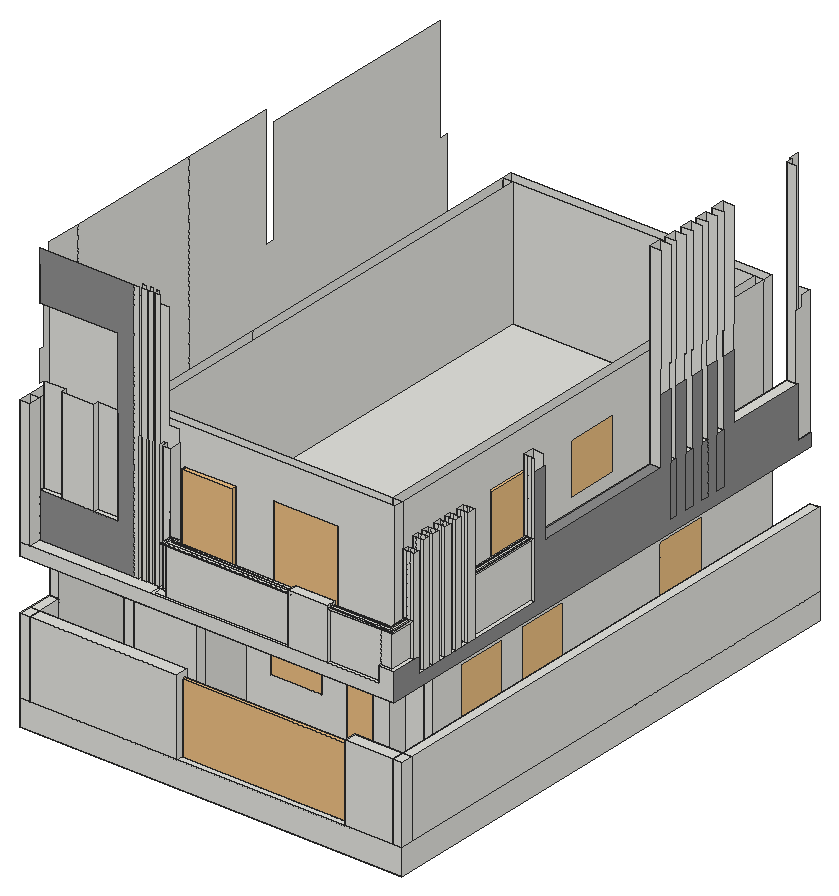
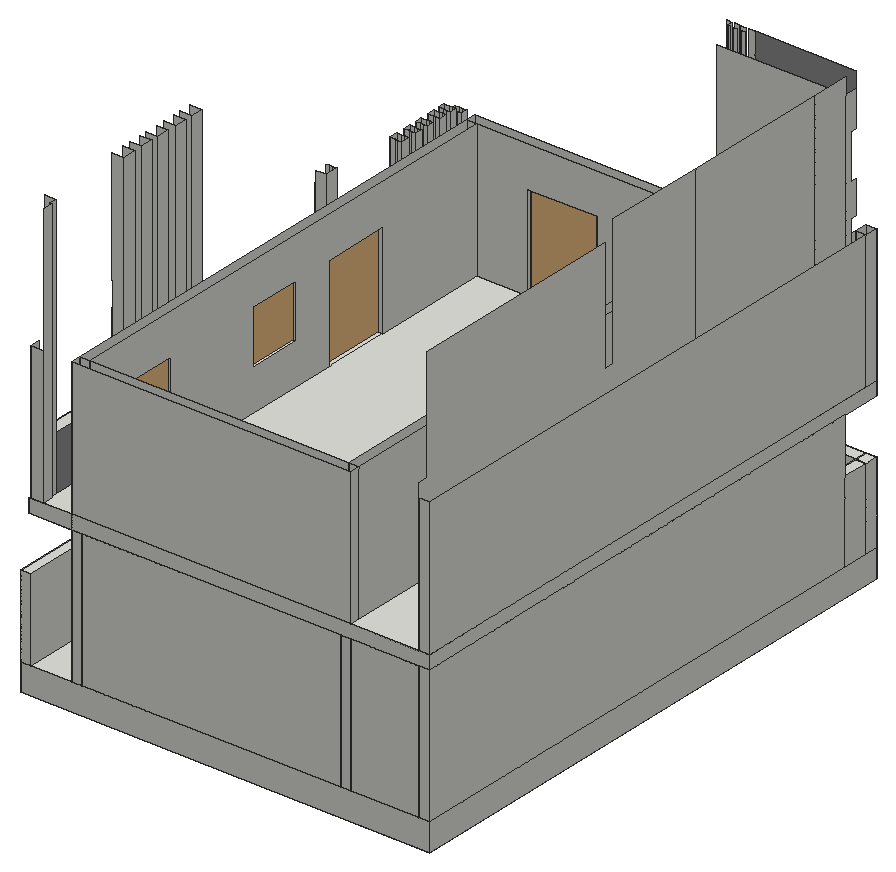
# SketchUp Ruby script. Lengths in inches.
U = 1.inch
M = Sketchup.active_model
def pt(a) = Geom::Point3d.new(a.map { |v| v * U })
def face(e, loops, mat)
  f = e.add_face(loops[0].map { |a| pt(a) })
  loops[1..].each { |l| e.add_face(l.map { |a| pt(a) }).erase! }
  f.material = f.back_material = mat if mat
  f
end
# faces: each face lists its corners as indices into pts; further lists are holes
def faces(e, pts, list, mat = nil) = list.each { |f| face(e, (f[0].is_a?(Array) ? f : [f]).map { |l| l.map { |i| pts[i] } }, mat) }
# xy, xz, yz: faces in a plane at the given z, y or x. An outline is a flat list of corners, or four numbers for a rectangle; further outlines are holes
def ring(l) = l.size == 4 ? [[l[0], l[1]], [l[2], l[1]], [l[2], l[3]], [l[0], l[3]]] : l.each_slice(2).to_a
def flat(e, list, mat, &to3) = list.each { |f| face(e, (f[0].is_a?(Array) ? f : [f]).map { |l| ring(l).map { |u, v| to3.(u, v) } }, mat) }
def xy(e, z, list, mat = nil) = flat(e, list, mat) { |x, y| [x, y, z] }
def xz(e, y, list, mat = nil) = flat(e, list, mat) { |x, z| [x, y, z] }
def yz(e, x, list, mat = nil) = flat(e, list, mat) { |y, z| [x, y, z] }
def lines(e, pts, list) = list.each { |a, b| e.add_line(pt(pts[a]), pt(pts[b])) }
# prism: a flat outline (further loops are holes) pulled along v
def prism(e, loops, v, mat = nil)
  f = face(e, loops, mat); d = Geom::Vector3d.new(v.map { |x| x * U })
  f.pushpull(f.normal.samedirection?(d) ? d.length : -d.length)
end
def box(e, o, s, mat = nil) = prism(e, [[o, [o[0] + s[0], o[1], o[2]], [o[0] + s[0], o[1] + s[1], o[2]], [o[0], o[1] + s[1], o[2]]]], [0, 0, s[2]], mat)
def at(x, y, z, deg = 0) = Geom::Transformation.translation(pt([x, y, z])) * Geom::Transformation.rotation(ORIGIN, Z_AXIS, deg.degrees)
def axes(o, x, y, z) = Geom::Transformation.new([*x, 0, *y, 0, *z, 0, *pt(o).to_a, 1])
def part(name) = M.definitions.add(name)
# library, detail: a bought-in or finely detailed component or shape, given as its bounding box
def library(name, o, s) = part(name).tap { |d| box(d.entities, o, s) }
def detail(e, o, s) = box(e.add_group.entities, o, s)
def put(e, d, t, mat = nil) = e.add_instance(d, t).tap { |i| i.material = mat if mat }
def group(e, t, mat = nil) = e.add_group.tap { |g| g.transformation = t; g.material = mat if mat }.entities
root = M.entities
M.materials.add("[Color M04]").color = [142, 142, 142]
c1 = library("Garage Gate 243 111",[-105.76,-3.7,0],[211.52,7.4,101.23])
c2 = library("Door 243 053",[-21.6,-2.79,-0.07],[43.2,5.58,82.64])
c3 = library("Window 46-15",[-34.06,-3.13,0],[68.12,6.24,59.06])
xy(root,-24,[[0,0,360,491.75]])
xy(root,0,[[0,0,9,11.75],[9,0,148.02,11.75],[148.02,0,306,11.75],[306,0,351,11.75],[351,0,360,11.75],
  [0,11.75,9,34.28],[[9,11.75,351,11.75,351,491.75,315,491.75,315,92.75,282,92.75,282,101.75,234,101.75,234,92.75,138,92.75,138,35.75,69,35.75,69,482.75,9,482.75,9,272.81,57,272.81,57,260.81,9,260.81],[320.75,14.17,337.0625,31.92]],[351,11.75,360,491.75],[320.75,14.17,337.0625,31.92],[0,34.28,9,491.75],
  [69,35.75,78,482.75],[78,35.75,138,44.75],[78,44.75,129,44.75,129,101.75,306,101.75,306,482.75,78,482.75],[129,44.75,138,101.75],[129,44.75,138,44.75,138,92.75,234,92.75,234,101.75,129,101.75],
  [138,92.75,234,101.75],[282,92.75,306,101.75],[306,92.75,315,125.75],[306,125.75,315,173.75],[306,173.75,315,491.75],
  [9,260.81,57,272.81],[9,482.75,69,491.75],[69,482.75,78,491.75],[78,482.75,306,491.75]])
xy(root,12,[[9,260.81,57,272.81]])
xy(root,18,[[9,248.81,57,260.81]])
xy(root,24,[[9,236.81,57,248.81]])
xy(root,30,[[9,224.81,57,236.81]])
xy(root,36,[[162,92.75,210,101.75],[306,197.75,315,245.75],[9,212.81,57,224.81],[306,359.75,315,407.75]])
xy(root,42,[[9,200.81,57,212.81]])
xy(root,48,[[9,188.81,57,200.81]])
xy(root,54,[[9,176.81,57,188.81]])
xy(root,60,[[9,164.81,57,176.81]])
xy(root,66,[[9,152.81,57,164.81]])
xy(root,72,[[0,0,9,11.75],[9,0,148.02,11.75],[306,0,351,11.75],[351,0,360,11.75],[0,11.75,9,34.28],
  [351,11.75,360,491.75],[9,140.81,57,152.81]])
xy(root,78,[[9,128.81,57,140.81]])
xy(root,84,[[162,92.75,210,101.75],[234,92.75,282,101.75],[9,116.81,57,128.81],[306,125.75,315,173.75],[306,197.75,315,245.75],
  [306,359.75,315,407.75]])
xy(root,90,[[9,104.81,57,116.81]])
xy(root,96,[[9,92.81,57,104.81]])
xy(root,102,[[9,80.81,57,92.81]])
xy(root,108,[[9,68.81,57,80.81]])
xy(root,114,[[9,56.81,57,68.81]])
xy(root,120,[[0,0,9,34.28],[9,0,9,34.28,57,34.28,57,56.81,69,56.81,69,0],[69,0,78,35.75],[[78,0,78,35.75,138,35.75,138,92.75,315,92.75,315,491.75,352.3125,491.75,352.3125,0],[320.75,14.17,337.0625,31.92]],[0,34.28,9,491.75],
  [9,34.28,57,56.81],[69,35.75,78,482.75],[78,35.75,138,44.75],[78,44.75,78,482.75,306,482.75,306,101.75,129,101.75,129,44.75],[129,44.75,138,101.75],
  [129,44.75,138,101.75],[138,92.75,306,101.75],[306,92.75,315,491.75],[9,187.47,69,482.75],[9,482.75,69,491.75],
  [69,482.75,78,491.75],[78,482.75,306,491.75]])
xy(root,132,[[0,0,9,11.75],[9,0,122.25,0,122.25,11.75,117.62,11.75,117.62,16.5625,115.5625,16.5625,115.5625,11.75,111.75,11.75,111.75,16.5625,109.5,16.5625,109.5,11.75,105.0625,11.75,105.0625,16.5625,102.625,16.5625,102.625,11.75,9,11.75],[122.25,0,252.63,0,252.63,2.7,124.95,2.7,124.95,9.05,122.25,9.05],[252.63,0,289.55,9.22],[289.55,0,337.97,2.7],
  [124.95,2.7,135.07,9.05],[135.07,2.7,135.07,9.05,138.35,9.14,138.35,5.97,252.63,5.97,252.63,2.7],[289.55,2.7,337.97,5.97],[138.35,5.97,252.63,5.97,252.63,9.22,141.6,9.22,138.35,9.14],[289.55,5.97,337.97,9.22],
  [122.25,9.05,135.07,9.05,138.35,9.14,141.6,9.22,341.78,9.22,341.78,482.53,339.69,482.53,339.69,491.75,315,491.75,315,220,306,220,306,160,315,160,315,47.75,261,47.75,261,56.75,201,56.75,201,47.75,165,47.75,165,56.75,117,56.75,117,47.75,69,47.75,69,56.81,9,56.81,9,22.5,132.375,22.5,132.375,11.75,125.16,11.75,125.16,16.5625,122.25,16.5625],[0,11.75,9,491.75],[9,11.75,9,22.5,132.375,22.5,132.375,11.75,125.16,11.75,125.16,16.5625,122.25,16.5625,122.25,11.75,117.62,11.75,117.62,16.5625,115.5625,16.5625,115.5625,11.75,111.75,11.75,111.75,16.5625,109.5,16.5625,109.5,11.75,105.0625,11.75,105.0625,16.5625,102.625,16.5625,102.625,11.75],[341.78,28.93,345.03,35.09],[345.03,28.93,348.3,35.09],
  [348.3,28.93,352.3125,35.09],[341.78,35.09,352.3125,41.08],[341.78,41.08,345.03,46.18],[345.03,41.08,348.3,46.18],[348.3,41.08,352.3125,46.18],
  [341.78,46.18,352.3125,52.82],[69,47.75,117,56.75],[165,47.75,201,56.75],[261,47.75,315,56.75],[341.78,52.82,345.03,60.24],
  [345.03,52.82,348.3,60.24],[348.3,52.82,352.3125,60.24],[69,56.75,78,482.75],[78,56.75,306,482.75],[306,56.75,315,160],
  [341.78,60.24,352.3125,66.7],[341.78,66.7,345.03,73.23],[345.03,66.7,348.3,73.23],[348.3,66.7,352.3125,73.23],[341.78,73.23,352.3125,79.37],
  [341.78,79.37,345.03,87.35],[345.03,79.37,348.3,87.35],[348.3,79.37,352.3125,87.35],[341.78,87.35,352.3125,94.89],[341.78,94.89,345.03,166.56],
  [345.03,94.89,348.3,166.56],[348.3,94.89,352.3125,166.56],[9,187.47,69,491.75],[306,220,315,482.75],[341.78,325.96,352.3125,332.62],
  [341.78,343.76,352.3125,351.72],[341.78,362.89,352.3125,369.53],[341.78,380.51,352.3125,388.24],[341.78,475.81,341.78,482.53,339.69,482.53,339.69,491.75,351,491.75,351,475.81],[351,475.81,352.3125,491.75],
  [69,482.75,315,491.75]])
xy(root,146.25,[[337.97,0,352.3125,0,352.3125,23.68,348.3,23.68,348.3,2.7,337.97,2.7],[337.97,2.7,337.97,5.97,345.03,5.97,345.03,23.68,348.3,23.68,348.3,2.7],[337.97,5.97,345.03,5.97,345.03,23.68,341.78,23.68,341.78,9.22,337.97,9.22],[341.78,23.68,352.3125,28.93]])
xy(root,168,[[306,256,315,304],[306,393.91,315,441.91]])
xy(root,173.74,[[9,11.75,29.4,16.5625],[60.19,11.75,82.8125,16.5625]])
xy(root,176.5,[[[132.625,0.25,132.625,11.4375,140.79,11.64,140.79,8.42,255.08,8.42,255.08,0.25],[135.07,2.7,252.63,2.7,252.63,5.97,138.35,5.97,138.35,9.14,135.07,9.05]],[[287.82,0.96,287.82,7.7,343.3,7.7,343.3,25.41,350.04,25.41,350.04,0.96],[289.55,2.7,348.3,2.7,348.3,23.68,345.03,23.68,345.03,5.97,289.55,5.97]],[135.07,2.7,135.07,9.05,138.35,9.14,138.35,5.97,252.63,5.97,252.63,2.7],[289.55,2.7,289.55,5.97,345.03,5.97,345.03,23.68,348.3,23.68,348.3,2.7]])
xy(root,177.8125,[[[132.625,0.25,255.08,0.25,255.08,8.42,140.79,8.42,140.79,11.64,132.625,11.4375],[135.07,2.7,135.07,9.05,138.35,9.14,138.35,5.97,252.63,5.97,252.63,2.7]],[[287.82,0.96,350.04,0.96,350.04,25.41,343.3,25.41,343.3,7.7,287.82,7.7],[289.55,2.7,289.55,5.97,345.03,5.97,345.03,23.68,348.3,23.68,348.3,2.7]],[135.07,2.7,252.63,2.7,252.63,5.97,138.35,5.97,138.35,9.14,135.07,9.05],[289.55,2.7,348.3,2.7,348.3,23.68,345.03,23.68,345.03,5.97,289.55,5.97]])
xy(root,180,[[252.63,0,289.55,9.22],[341.78,325.96,352.3125,332.62],[341.78,343.76,352.3125,351.72],[341.78,362.89,352.3125,369.53],[341.78,380.51,352.3125,388.24],
  [341.78,401.04,352.3125,475.81]])
xy(root,180,[[341.78,177.375,352.3125,314.875]],"[Color M04]")
xy(root,183.4375,[[[343.49,93.36,349.84,168.09],[345.03,94.89,348.3,166.56]],[345.03,94.89,348.3,166.56]])
xy(root,184.75,[[[343.49,93.36,349.84,168.09],[345.03,94.89,348.3,166.56]],[345.03,94.89,348.3,166.56]])
xz(root,0,[[0,-24,360,0],[0,0,9,72],[9,0,148.02,72],[306,0,351,72],[351,0,360,72],
  [0,120,352.3125,120,352.3125,146.25,337.97,146.25,337.97,132,0,132],[0,132,9,252],[252.63,132,289.55,180]])
xz(root,0.25,[[132.625,176.5,255.08,177.8125]])
xz(root,0.96,[[287.82,176.5,337.97,177.8125],[337.97,176.5,350.04,177.8125]])
xz(root,2.7,[[135.07,132,252.63,176.5],[289.55,132,337.97,176.5],[337.97,146.25,348.3,176.5],[135.07,176.5,252.63,177.8125],[289.55,176.5,337.97,177.8125],
  [337.97,176.5,348.3,177.8125]])
xz(root,5.97,[[138.35,132,252.63,176.5],[289.55,132,337.97,176.5],[337.97,146.25,345.03,176.5],[138.35,176.5,252.63,177.8125],[289.55,176.5,337.97,177.8125],
  [337.97,176.5,345.03,177.8125]])
xz(root,7.7,[[287.82,176.5,337.97,177.8125],[337.97,176.5,343.3,177.8125]])
xz(root,8.42,[[140.79,176.5,255.08,177.8125]])
xz(root,9.22,[[252.63,132,289.55,180],[337.97,132,341.78,146.25]])
xz(root,11.75,[[0,0,9,72],[9,0,148.02,72],[306,0,351,72],[351,0,360,72],[0,132,9,252],
  [97.8125,132,102.625,378.375],[105.0625,132,109.5,378.375],[111.75,132,115.5625,378.375],[117.62,132,122.25,378.375],[125.16,132,130.91,132,131.25,252,125.16,252],
  [130.91,132,132.375,132,132.375,252,131.25,252],[29.4,173.74,60.19,264]])
xz(root,11.75,[[9,132,97.8125,132,97.8125,378.375,9,378.375,9,332.24,82.8125,332.24,82.8125,173.74,9,173.74]],"[Color M04]")
xz(root,14.17,[[320.75,0,337.0625,120]])
xz(root,16.5625,[[102.625,132,105.0625,378.375],[109.5,132,111.75,378.375],[115.5625,132,117.62,378.375],[122.25,132,125.16,252],[9,173.74,29.4,264],
  [60.19,173.74,82.8125,264]])
xz(root,22.5,[[9,132,9,363.8125,122.25,363.8125,122.25,264,131.25,264,131.25,252,132.375,252,132.375,132]])
xz(root,23.68,[[341.78,146.25,345.03,235.625],[345.03,146.25,348.3,176.5],[348.3,146.25,352.3125,235.625],[345.03,176.5,348.3,177.8125],[345.03,177.8125,348.3,235.625]])
xz(root,25.41,[[343.3,176.5,350.04,177.8125]])
xz(root,28.93,[[341.78,132,345.03,146.25],[345.03,132,348.3,146.25],[348.3,132,352.3125,146.25],[341.78,146.25,345.03,235.625],[345.03,146.25,348.3,235.625],
  [348.3,146.25,352.3125,235.625]])
xz(root,31.92,[[320.75,0,337.0625,120]])
xz(root,34.28,[[0,0,9,72],[0,72,9,120]])
xz(root,35.09,[[341.78,132,345.03,241.9375],[345.03,132,348.3,241.9375],[348.3,132,352.3125,241.9375]])
xz(root,35.75,[[69,0,78,120],[78,0,138,120]])
xz(root,41.08,[[341.78,132,345.03,241.9375],[345.03,132,348.3,241.9375],[348.3,132,352.3125,241.9375]])
xz(root,44.75,[[78,0,129,120],[129,0,138,120]])
xz(root,46.18,[[341.78,132,345.03,241.9375],[345.03,132,348.3,241.9375],[348.3,132,352.3125,241.9375]])
xz(root,47.75,[[69,132,117,132,117,216,165,216,165,132,201,132,201,216,261,216,261,132,315,132,315,252,69,252]])
xz(root,52.82,[[341.78,132,345.03,241.9375],[345.03,132,348.3,241.9375],[348.3,132,352.3125,241.9375]])
xz(root,56.75,[[69,132,78,252],[78,132,78,252,306,252,306,132,261,132,261,216,201,216,201,132,165,132,165,216,117,216,117,132],[306,132,315,252]])
xz(root,56.81,[[9,114,57,120],[9,120,69,132]])
xz(root,60.24,[[341.78,132,345.03,241.9375],[345.03,132,348.3,241.9375],[348.3,132,352.3125,241.9375]])
xz(root,66.7,[[341.78,132,345.03,241.9375],[345.03,132,348.3,241.9375],[348.3,132,352.3125,241.9375]])
xz(root,68.81,[[9,108,57,114]])
xz(root,73.23,[[341.78,132,345.03,241.9375],[345.03,132,348.3,241.9375],[348.3,132,352.3125,241.9375]])
xz(root,79.37,[[341.78,132,345.03,241.9375],[345.03,132,348.3,241.9375],[348.3,132,352.3125,241.9375]])
xz(root,80.81,[[9,102,57,108]])
xz(root,87.35,[[341.78,132,345.03,241.9375],[345.03,132,348.3,241.9375],[348.3,132,352.3125,241.9375]])
xz(root,92.75,[[[138,0,234,0,234,84,282,84,282,0,306,0,306,120,138,120],[162,36,210,84]],[306,0,315,120]])
xz(root,92.81,[[9,96,57,102]])
xz(root,93.36,[[343.49,183.4375,349.84,184.75]])
xz(root,94.89,[[341.78,132,345.03,241.9375],[345.03,132,348.3,183.4375],[348.3,132,352.3125,241.9375],[345.03,183.4375,348.3,184.75],[345.03,184.75,348.3,241.9375]])
xz(root,101.75,[[129,0,138,120],[[138,0,138,120,306,120,306,0,282,0,282,84,234,84,234,0],[162,36,210,84]]])
xz(root,104.81,[[9,90,57,96]])
xz(root,116.81,[[9,84,57,90]])
xz(root,125.75,[[306,0,315,84]])
xz(root,128.81,[[9,78,57,84]])
xz(root,140.81,[[9,72,57,78]])
xz(root,152.81,[[9,66,57,72]])
xz(root,160,[[306,132,315,216]])
xz(root,164.81,[[9,60,57,66]])
xz(root,166.56,[[341.78,132,345.03,252.9375],[345.03,132,348.3,183.4375],[348.3,132,352.3125,132,352.3125,241.9375,351,241.9375,351,252,348.3,252.9375],[345.03,183.4375,348.3,184.75],[345.03,184.75,348.3,252.9375]])
xz(root,168.09,[[343.49,183.4375,349.84,184.75]])
xz(root,173.75,[[306,0,315,84]])
xz(root,176.81,[[9,54,57,60]])
xz(root,177.375,[[341.78,180,341.78,252.9375,351,252,351,241.9375,352.3125,241.9375,352.3125,180]])
xz(root,187.47,[[9,120,69,132]])
xz(root,188.81,[[9,48,57,54]])
xz(root,197.75,[[306,36,315,84]])
xz(root,200.81,[[9,42,57,48]])
xz(root,212.81,[[9,36,57,42]])
xz(root,220,[[306,132,315,216]])
xz(root,224.81,[[9,30,57,36]])
xz(root,236.81,[[9,24,57,30]])
xz(root,245.75,[[306,36,315,84]])
xz(root,248.81,[[9,18,57,24]])
xz(root,256,[[306,168,315,216]])
xz(root,260.81,[[9,12,57,18]])
xz(root,272.81,[[9,0,57,12]])
xz(root,304,[[306,168,315,216]])
xz(root,314.875,[[341.78,180,352.3125,180,352.3125,241.9375,351,241.9375,351,264,352.3125,264,352.3125,363.8125,341.78,363.8125]])
xz(root,325.96,[[341.78,132,352.3125,180],[341.78,180,341.78,363.8125,352.3125,363.8125,352.3125,264,351,264,351,241.9375,352.3125,241.9375,352.3125,180]])
xz(root,332.62,[[341.78,132,352.3125,180],[341.78,180,352.3125,180,352.3125,241.9375,351,241.9375,351,264,352.3125,264,352.3125,363.8125,341.78,363.8125]])
xz(root,343.76,[[341.78,132,352.3125,180],[341.78,180,341.78,363.8125,352.3125,363.8125,352.3125,264,351,264,351,241.9375,352.3125,241.9375,352.3125,180]])
xz(root,351.72,[[341.78,132,352.3125,180],[341.78,180,352.3125,180,352.3125,241.9375,351,241.9375,351,264,352.3125,264,352.3125,363.8125,341.78,363.8125]])
xz(root,359.75,[[306,36,315,84]])
xz(root,362.89,[[341.78,132,352.3125,180],[341.78,180,341.78,363.8125,352.3125,363.8125,352.3125,264,351,264,351,241.9375,352.3125,241.9375,352.3125,180]])
xz(root,369.53,[[341.78,132,352.3125,180],[341.78,180,352.3125,180,352.3125,241.9375,351,241.9375,351,264,352.3125,264,352.3125,363.8125,341.78,363.8125]])
xz(root,380.51,[[341.78,132,352.3125,180],[341.78,180,341.78,363.8125,352.3125,363.8125,352.3125,264,351,264,351,241.9375,352.3125,241.9375,352.3125,180]])
xz(root,388.24,[[341.78,132,352.3125,180],[341.78,180,352.3125,180,352.3125,241.9375,351,241.9375,351,264,352.3125,264,352.3125,363.8125,341.78,363.8125]])
xz(root,393.91,[[306,168,315,216]])
xz(root,401.04,[[341.78,180,341.78,363.8125,352.3125,363.8125,352.3125,264,351,264,351,241.9375,352.3125,241.9375,352.3125,180]])
xz(root,407.75,[[306,36,315,84]])
xz(root,441.91,[[306,168,315,216]])
xz(root,475.81,[[341.78,132,351,180],[351,132,352.3125,180],[341.78,180,351,363.8125]])
xz(root,482.53,[[339.69,132,341.78,363.8125]])
xz(root,482.75,[[9,0,69,120],[69,0,78,120],[78,0,306,120],[69,132,78,252],[78,132,306,252],
  [306,132,315,252]])
xz(root,491.75,[[0,-24,360,0],[0,0,9,120],[9,0,69,120],[69,0,78,120],[78,0,306,120],
  [306,0,315,120],[351,0,360,72],[0,120,315,132],[315,120,352.3125,132],[0,132,9,252],
  [69,132,315,252],[339.69,132,351,252]])
yz(root,0,[[0,-24,491.75,0],[0,0,11.75,72],[11.75,0,34.28,72],[34.28,0,491.75,120],[0,120,491.75,132],
  [0,132,11.75,252],[11.75,132,491.75,252]])
yz(root,9,[[0,0,11.75,72],[11.75,0,34.28,72],[260.81,0,34.28,120,56.81,120,56.81,114,68.81,114,68.81,108,80.81,108,80.81,102,92.81,102,92.81,96,104.81,96,104.81,90,116.81,90,116.81,84,128.81,84,128.81,78,140.81,78,140.81,72,152.81,72,152.81,66,164.81,66,164.81,60,176.81,60,176.81,54,188.81,54,188.81,48,200.81,48,200.81,42,212.81,42,212.81,36,224.81,36,224.81,30,236.81,30,236.81,24,248.81,24,248.81,18,260.81,18,260.81,12,272.81,12,272.81,0],[34.28,0,260.81,0,34.28,120],[272.81,0,482.75,0,482.75,120,56.81,120,56.81,114,68.81,114,68.81,108,80.81,108,80.81,102,92.81,102,92.81,96,104.81,96,104.81,90,116.81,90,116.81,84,128.81,84,128.81,78,140.81,78,140.81,72,152.81,72,152.81,66,164.81,66,164.81,60,176.81,60,176.81,54,188.81,54,188.81,48,200.81,48,200.81,42,212.81,42,212.81,36,224.81,36,224.81,30,236.81,30,236.81,24,248.81,24,248.81,18,260.81,18,260.81,12,272.81,12],
  [482.75,0,491.75,120],[56.81,120,187.47,132],[0,132,11.75,252],[11.75,132,22.5,132,22.5,363.8125,11.75,363.8125,11.75,332.24,16.5625,332.24,16.5625,292.85,11.75,292.85,11.75,264,16.5625,264,16.5625,173.74,11.75,173.74],[22.5,132,56.81,378.375],
  [56.81,132,187.47,378.375],[187.47,132,491.75,132,491.75,264,482.75,264,482.75,363.8125,287.1875,363.8125,287.1875,264,278.1875,264,278.1875,378.375,187.47,378.375],[11.75,173.74,16.5625,252]])
yz(root,29.4,[[11.75,173.74,16.5625,264]])
yz(root,57,[[260.81,0,272.81,0,272.81,12,260.81,12,260.81,18,248.81,18,248.81,24,236.81,24,236.81,30,224.81,30,224.81,36,212.81,36,212.81,42,200.81,42,200.81,48,188.81,48,188.81,54,176.81,54,176.81,60,164.81,60,164.81,66,152.81,66,152.81,72,140.81,72,140.81,78,128.81,78,128.81,84,116.81,84,116.81,90,104.81,90,104.81,96,92.81,96,92.81,102,80.81,102,80.81,108,68.81,108,68.81,114,56.81,114,56.81,120,34.28,120]])
yz(root,60.19,[[11.75,173.74,16.5625,264]])
yz(root,69,[[35.75,0,482.75,120],[482.75,0,491.75,120],[56.81,120,187.47,132],[47.75,132,56.75,252],[56.75,132,56.81,252],
  [56.81,132,187.47,252],[187.47,132,482.75,252],[482.75,132,491.75,252]])
yz(root,78,[[35.75,0,44.75,120],[44.75,0,482.75,120],[482.75,0,491.75,120],[56.75,132,482.75,252]])
yz(root,82.8125,[[11.75,173.74,16.5625,264]])
yz(root,102.625,[[11.75,132,16.5625,252]])
yz(root,105.0625,[[11.75,132,16.5625,252]])
yz(root,109.5,[[11.75,132,16.5625,252]])
yz(root,111.75,[[11.75,132,16.5625,252]])
yz(root,115.5625,[[11.75,132,16.5625,252]])
yz(root,117,[[47.75,132,56.75,216]])
yz(root,117.62,[[11.75,132,16.5625,378.375]])
yz(root,122.25,[[11.75,132,16.5625,252]])
yz(root,125.16,[[11.75,132,16.5625,252]])
yz(root,129,[[44.75,0,101.75,120]])
yz(root,132.375,[[11.75,132,22.5,252]])
yz(root,132.625,[[0.25,176.5,11.4375,177.8125]])
yz(root,135.07,[[2.7,132,9.05,176.5],[2.7,176.5,9.05,177.8125]])
yz(root,138,[[35.75,0,44.75,120],[44.75,0,92.75,120],[92.75,0,101.75,120]])
yz(root,138.35,[[5.97,132,9.14,176.5],[5.97,176.5,9.14,177.8125]])
yz(root,140.79,[[8.42,176.5,11.64,177.8125]])
yz(root,148.02,[[0,0,11.75,72]])
yz(root,162,[[92.75,36,101.75,84]])
yz(root,165,[[47.75,132,56.75,216]])
yz(root,201,[[47.75,132,56.75,216]])
yz(root,210,[[92.75,36,101.75,84]])
yz(root,234,[[92.75,0,101.75,84]])
yz(root,252.63,[[0,132,2.7,180],[2.7,132,5.97,176.5],[5.97,132,9.22,180],[2.7,176.5,5.97,177.8125],[2.7,177.8125,5.97,180]])
yz(root,255.08,[[0.25,176.5,8.42,177.8125]])
yz(root,261,[[47.75,132,56.75,216]])
yz(root,282,[[92.75,0,101.75,84]])
yz(root,287.82,[[0.96,176.5,7.7,177.8125]])
yz(root,289.55,[[0,132,2.7,180],[2.7,132,5.97,176.5],[5.97,132,9.22,180],[2.7,176.5,5.97,177.8125],[2.7,177.8125,5.97,180]])
yz(root,306,[[0,0,11.75,72],[92.75,0,101.75,120],[[101.75,0,101.75,120,482.75,120,482.75,0,173.75,0,173.75,84,125.75,84,125.75,0],[197.75,36,245.75,84],[359.75,36,407.75,84]],[482.75,0,491.75,120],[[56.75,132,56.75,252,482.75,252,482.75,132,220,132,220,216,160,216,160,132],[256,168,304,216],[393.91,168,441.91,216]]])
yz(root,315,[[[92.75,0,125.75,0,125.75,84,173.75,84,173.75,0,491.75,0,491.75,120,92.75,120],[197.75,36,245.75,84],[359.75,36,407.75,84]],[47.75,132,56.75,252],[[56.75,132,160,132,160,216,220,216,220,132,482.75,132,482.75,252,56.75,252],[256,168,304,216],[393.91,168,441.91,216]],[482.75,132,491.75,252]])
yz(root,320.75,[[14.17,0,31.92,120]])
yz(root,337.0625,[[14.17,0,31.92,120]])
yz(root,337.97,[[0,132,2.7,146.25],[2.7,132,5.97,146.25],[5.97,132,9.22,146.25]])
yz(root,339.69,[[482.53,132,491.75,363.8125]])
yz(root,341.78,[[9.22,132,23.68,146.25],[23.68,132,28.93,146.25],[35.09,132,41.08,241.9375],[46.18,132,52.82,241.9375],[60.24,132,66.7,241.9375],
  [73.23,132,79.37,241.9375],[87.35,132,94.89,241.9375],[166.56,132,177.375,252.9375],[314.875,132,325.96,363.8125],[325.96,132,332.62,180],
  [332.62,132,343.76,363.8125],[343.76,132,351.72,180],[351.72,132,362.89,363.8125],[362.89,132,369.53,180],[369.53,132,380.51,363.8125],
  [380.51,132,388.24,180],[388.24,132,401.04,363.8125],[475.81,132,482.53,363.8125],[23.68,146.25,28.93,235.625]])
yz(root,341.78,[[177.375,132,314.875,180],[401.04,132,475.81,180]],"[Color M04]")
yz(root,343.3,[[7.7,176.5,25.41,177.8125]])
yz(root,343.49,[[93.36,183.4375,168.09,184.75]])
yz(root,345.03,[[94.89,132,166.56,183.4375],[5.97,146.25,23.68,176.5],[5.97,176.5,23.68,177.8125],[94.89,183.4375,166.56,184.75]])
yz(root,348.3,[[94.89,132,166.56,183.4375],[2.7,146.25,23.68,176.5],[2.7,176.5,23.68,177.8125],[94.89,183.4375,166.56,184.75]])
yz(root,349.84,[[93.36,183.4375,168.09,184.75]])
yz(root,350.04,[[0.96,176.5,25.41,177.8125]])
yz(root,351,[[0,0,11.75,72],[11.75,0,491.75,72],[475.81,132,491.75,132,491.75,252,482.75,252,482.75,241.9375,475.81,241.9375]])
yz(root,352.3125,[[35.09,132,41.08,241.9375],[46.18,132,52.82,241.9375],[60.24,132,66.7,241.9375],[73.23,132,79.37,241.9375],[87.35,132,94.89,241.9375],
  [23.68,146.25,28.93,235.625]])
yz(root,352.3125,[[0,120,491.75,120,491.75,132,475.81,132,475.81,180,401.04,180,401.04,241.9375,388.24,241.9375,388.24,132,380.51,132,380.51,241.9375,369.53,241.9375,369.53,132,362.89,132,362.89,241.9375,351.72,241.9375,351.72,132,343.76,132,343.76,241.9375,332.62,241.9375,332.62,132,325.96,132,325.96,241.9375,314.875,241.9375,314.875,180,177.375,180,177.375,241.9375,166.56,241.9375,166.56,132,28.93,132,28.93,146.25,0,146.25],[325.96,132,332.62,180],[343.76,132,351.72,180],[362.89,132,369.53,180],[380.51,132,388.24,180]],"[Color M04]")
yz(root,360,[[0,-24,491.75,0],[0,0,11.75,72],[11.75,0,491.75,72]])
p = [[9,34.28,120],[9,260.81,0],[57,260.81,0],[57,34.28,120],[138.35,9.14,132],[135.07,9.05,132],
  [135.07,9.05,176.5],[138.35,9.14,176.5],[135.07,9.05,177.8125],[138.35,9.14,177.8125],[140.79,11.64,176.5],[132.625,11.4375,176.5],
  [132.625,11.4375,177.8125],[140.79,11.64,177.8125],[59.78,38.53,132],[59.78,47.59,132],[18.22,47.59,132],[18.22,31.72,132],
  [311.97,214.03,132],[311.97,165.97,132],[255.03,50.78,132],[206.97,50.78,132],[159.03,50.78,132],[122.97,50.78,132],
  [63.03,41.78,132],[63.03,50.84,132],[14.97,50.84,132],[14.97,28.47,132],[308.7,217.3,132],[308.7,162.7,132],
  [258.3,54.05,132],[203.7,54.05,132],[162.3,54.05,132],[119.7,54.05,132],[66.3,45.05,132],[66.3,54.11,132],
  [11.7,54.11,132],[11.7,25.2,132]]
faces(root,p,[[0,1,2,3],[4,5,6,7],[7,6,8,9],[10,11,12,13]])
lines(root,p,[[14,15],[15,16],[16,17],[18,19],[20,21],[22,23],[24,25],[25,26],[26,27],[28,29],[30,31],[32,33],
  [34,35],[35,36],[36,37]])
put(root,c1,axes([227.02,7.65,0],[0.74674,0,0],[0,0.46,0],[0,0,0.65]))
put(root,c2,axes([258,95.54,0.07],[-1.11105,0,0],[0,-1,0],[0,0,1.01657]))
put(root,c2,axes([312.21,149.75,0.07],[0,-1.11105,0],[1,0,0],[0,0,1.01657]))
put(root,c3,axes([186,95.88,36],[0.70474,0,0],[0,1,0],[0,0,0.8128]))
put(root,c3,axes([311.87,221.75,36],[0,0.70474,0],[-1,0,0],[0,0,0.8128]))
put(root,c3,axes([311.87,383.75,36],[0,0.70474,0],[-1,0,0],[0,0,0.8128]))
put(root,c3,axes([139.87,48.92,130.7],[0.70474,0,0],[0,1,0],[0,0,1.4224]))
put(root,c2,axes([313.56,190,131.43],[0,-1.38881,0],[1,0,0],[0,0,1.01657]))
put(root,c2,axes([231,50.54,132.07],[1.38881,0,0],[0,1,0],[0,0,1.01657]))
put(root,c3,axes([311.87,417.91,168],[0,0.70474,0],[-1,0,0],[0,0,0.8128]))
put(root,c3,axes([311.87,280,168],[0,0.70474,0],[-1,0,0],[0,0,0.8128]))
